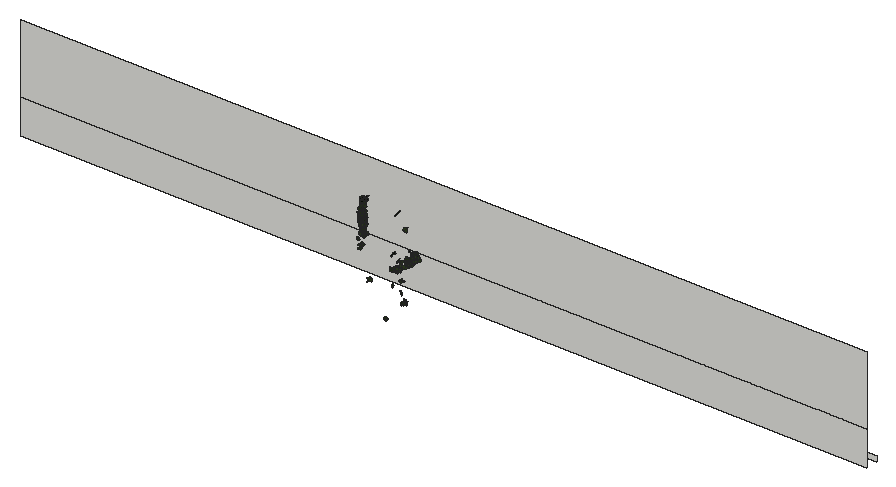
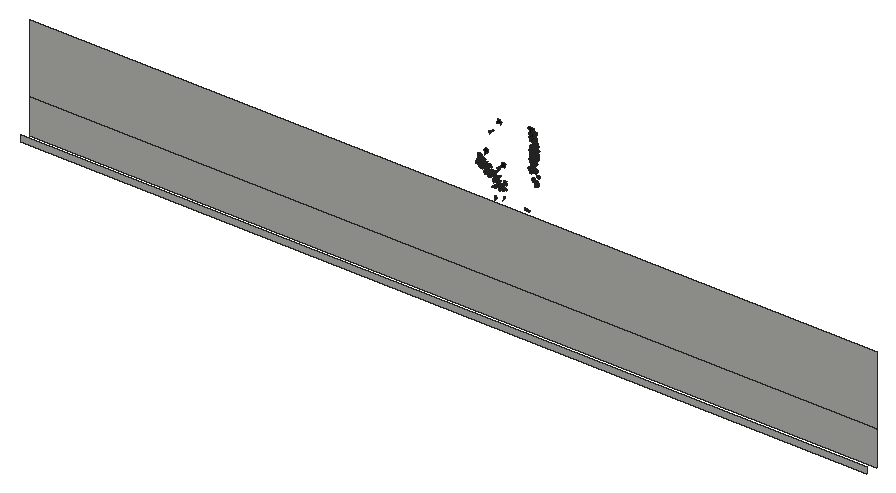
# SketchUp Ruby script. Lengths in inches.
U = 1.inch
M = Sketchup.active_model
def pt(a) = Geom::Point3d.new(a.map { |v| v * U })
def face(e, loops, mat)
  f = e.add_face(loops[0].map { |a| pt(a) })
  loops[1..].each { |l| e.add_face(l.map { |a| pt(a) }).erase! }
  f.material = f.back_material = mat if mat
  f
end
# faces: each face lists its corners as indices into pts; further lists are holes
def faces(e, pts, list, mat = nil) = list.each { |f| face(e, (f[0].is_a?(Array) ? f : [f]).map { |l| l.map { |i| pts[i] } }, mat) }
# xy, xz, yz: faces in a plane at the given z, y or x. An outline is a flat list of corners, or four numbers for a rectangle; further outlines are holes
def ring(l) = l.size == 4 ? [[l[0], l[1]], [l[2], l[1]], [l[2], l[3]], [l[0], l[3]]] : l.each_slice(2).to_a
def flat(e, list, mat, &to3) = list.each { |f| face(e, (f[0].is_a?(Array) ? f : [f]).map { |l| ring(l).map { |u, v| to3.(u, v) } }, mat) }
def xy(e, z, list, mat = nil) = flat(e, list, mat) { |x, y| [x, y, z] }
def xz(e, y, list, mat = nil) = flat(e, list, mat) { |x, z| [x, y, z] }
def yz(e, x, list, mat = nil) = flat(e, list, mat) { |y, z| [x, y, z] }
def lines(e, pts, list) = list.each { |a, b| e.add_line(pt(pts[a]), pt(pts[b])) }
# prism: a flat outline (further loops are holes) pulled along v
def prism(e, loops, v, mat = nil)
  f = face(e, loops, mat); d = Geom::Vector3d.new(v.map { |x| x * U })
  f.pushpull(f.normal.samedirection?(d) ? d.length : -d.length)
end
def box(e, o, s, mat = nil) = prism(e, [[o, [o[0] + s[0], o[1], o[2]], [o[0] + s[0], o[1] + s[1], o[2]], [o[0], o[1] + s[1], o[2]]]], [0, 0, s[2]], mat)
def at(x, y, z, deg = 0) = Geom::Transformation.translation(pt([x, y, z])) * Geom::Transformation.rotation(ORIGIN, Z_AXIS, deg.degrees)
def axes(o, x, y, z) = Geom::Transformation.new([*x, 0, *y, 0, *z, 0, *pt(o).to_a, 1])
def part(name) = M.definitions.add(name)
# library, detail: a bought-in or finely detailed component or shape, given as its bounding box
def library(name, o, s) = part(name).tap { |d| box(d.entities, o, s) }
def detail(e, o, s) = box(e.add_group.entities, o, s)
def put(e, d, t, mat = nil) = e.add_instance(d, t).tap { |i| i.material = mat if mat }
def group(e, t, mat = nil) = e.add_group.tap { |g| g.transformation = t; g.material = mat if mat }.entities
root = M.entities
M.materials.add("1026 AP 7946 SUNNY SIDE UP").color = [254, 231, 186]
M.materials.add("efeu1").color = [18, 25, 13]
M.materials.add("efeu2").color = [43, 57, 29]
c1 = part("ivyleaf_10")
p = [[0,0.5,-0.03],[-0.0625,2.02,-0.43],[-0.19,2.01,-0.46],[-0.54,1.05,-0.29],[-0.52,0.625,-0.18],[-0.83,0.76,-0.28],
  [-1.16,0.64,-0.33],[-1.15,0.33,-0.24],[-0.77,-0.39,0.02],[-0.3,-0.51,0.16],[0.04,-0.48,0.23],[-0.02,2.01,-0.4375],
  [-0.06,2.01,-0.43],[0.04,-0.49,0.23],[0.67,-0.49,0.14],[1.38,0.36,-0.2],[1.375,0.51,-0.24],[0.81,0.65,-0.19],
  [0.62,0.59,-0.15],[0.6,1.09,-0.28],[0.5,1.23,-0.31]]
faces(c1.entities,p,[[0,1,2,3,4,5,6,7,8,9,10],[11,12,0,13,14,15,16,17,18,19,20]],"efeu2")
c2 = part("ivyleaf_9")
p = [[1.54,2.16,1.25],[1.36,2.04,1.19],[-0.21,0.99,0.68],[-0.71,1.11,0.82],[-0.85,0.86,0.67],[-0.8,0.17,0.21],
  [-0.9,-0.01,0.1],[-0.67,-0.16,-0.02],[-0.08,-0.08,-0.05],[-0.03,-0.6,-0.4],[0.65,-0.88,-0.66],[0.83,-0.6,-0.49],
  [1.29,-0.42,-0.43],[1.8125,-0.07,-0.26],[1.21,0.44,0.15]]
faces(c2.entities,p,[[0,1,2,3,4,5,6,7,8,9,10,11,12,13,14]],"efeu1")
xz(root,227,[[30,246,177,252],[30,252,177,264]])
xz(root,229,[[30,246,177,247]])
put(root,c1,axes([99.8,213.53,264.95],[-0.08573,0.18101,-0.009],[-0.00321,-0.0117,-0.20128],[-0.3078,-0.05029,0.0046]),"1026 AP 7946 SUNNY SIDE UP")
put(root,c1,axes([99.82,213.11,265.17],[-0.13525,0.17041,-0.00934],[-0.00346,-0.01302,-0.20142],[-0.28985,-0.07936,0.00676]),"1026 AP 7946 SUNNY SIDE UP")
put(root,c1,axes([99.62,213.2,260.61],[0.00688,-0.00404,0.19077],[0.29489,-0.04004,-0.00576],[0.06813,0.17374,0.00566]),"1026 AP 7946 SUNNY SIDE UP")
put(root,c1,axes([99.73,213.47,263.92],[0.09541,0.05576,-0.17419],[0.16528,0.13172,0.08579],[0.2421,-0.1119,0.01008]),"1026 AP 7946 SUNNY SIDE UP")
put(root,c1,axes([99.8125,213.33,263.53],[0.16968,0.1463,-0.03606],[-0.01785,-0.03583,-0.18981],[-0.25497,0.09987,-0.0107]),"1026 AP 7946 SUNNY SIDE UP")
put(root,c1,axes([100.1,213.17,263.67],[-0.03089,0.023,0.19132],[-0.29433,0.04551,-0.02458],[-0.08132,-0.17346,0.01629]),"1026 AP 7946 SUNNY SIDE UP")
put(root,c1,axes([100,213.125,264.22],[0.18705,-0.12329,-0.09138],[-0.10102,0.05909,-0.17613],[0.23196,0.12515,-0.00302]),"1026 AP 7946 SUNNY SIDE UP")
put(root,c1,axes([99.92,213.55,265.11],[-0.22966,-0.12001,-0.04682],[0.08561,0.00591,-0.19115],[0.19823,-0.14159,0.0283]),"1026 AP 7946 SUNNY SIDE UP")
put(root,c1,axes([99.96,213.55,264.52],[0.00212,0.17404,0.05604],[-0.07134,0.04899,-0.18048],[-0.29904,-0.01045,0.04345]),"1026 AP 7946 SUNNY SIDE UP")
put(root,c1,axes([99.96,213.58,263.82],[0.14893,-0.15282,0.01887],[0.00536,-0.02078,-0.18876],[0.26148,0.08746,-0.00687]),"1026 AP 7946 SUNNY SIDE UP")
put(root,c1,axes([99.98,213.3125,263.88],[0.0121,0.13669,-0.11707],[-0.05804,-0.10803,-0.14612],[-0.29336,0.02701,0.02408]),"1026 AP 7946 SUNNY SIDE UP")
put(root,c1,axes([100.11,213.24,263.96],[-0.23706,0.08116,0.09126],[-0.16438,-0.00676,-0.16509],[-0.11128,-0.16292,0.04947]),"1026 AP 7946 SUNNY SIDE UP")
put(root,c1,axes([99.96,213.56,263.99],[0.01126,0.15169,0.10111],[-0.01801,0.09271,-0.1607],[-0.30103,0.00013,0.0134]),"1026 AP 7946 SUNNY SIDE UP")
put(root,c1,axes([100.09,213.17,263.96],[0.26296,-0.01763,-0.10344],[-0.16562,-0.01098,-0.16586],[0.01547,0.18212,-0.01744]),"1026 AP 7946 SUNNY SIDE UP")
put(root,c1,axes([99.98,213.55,265.05],[0.0413,0.18007,-0.03465],[-0.03651,-0.03197,-0.19415],[-0.30916,0.02783,0.0183]),"1026 AP 7946 SUNNY SIDE UP")
put(root,c1,axes([99.96,213.3125,264.65],[-0.21143,-0.10896,-0.08139],[0.10849,0.04001,-0.17622],[0.19617,-0.13956,0.00973]),"1026 AP 7946 SUNNY SIDE UP")
put(root,c1,axes([100.05,213.16,264.73],[-0.29522,-0.07091,0.01055],[-0.00665,-0.01883,-0.2006],[0.12158,-0.17322,0.01464]),"1026 AP 7946 SUNNY SIDE UP")
put(root,c1,axes([100.01,213.58,265.22],[0.2454,-0.11687,0.00366],[-0.00906,-0.01445,-0.1986],[0.19836,0.14392,-0.01361]),"1026 AP 7946 SUNNY SIDE UP")
put(root,c1,axes([100.05,213.1875,264.34],[0.21336,-0.13975,-0.01992],[-0.03616,0.00335,-0.20065],[0.23618,0.12676,-0.01273]),"1026 AP 7946 SUNNY SIDE UP")
put(root,c1,axes([99.99,213.13,259.1],[-0.13186,-0.14776,0.0643],[0.03866,0.05801,0.17939],[-0.26924,0.08069,-0.00573]),"1026 AP 7946 SUNNY SIDE UP")
put(root,c1,axes([99.84,213.53,263.92],[-0.07983,-0.0293,0.18382],[0.26154,0.07681,0.06015],[-0.1393,0.16101,0.00759]),"1026 AP 7946 SUNNY SIDE UP")
put(root,c1,axes([100.16,213.22,263.12],[0.16699,-0.05763,-0.14715],[-0.1384,0.11603,-0.11356],[0.21039,0.12207,0.04209]),"1026 AP 7946 SUNNY SIDE UP")
put(root,c1,axes([99.92,213.3,262.71],[-0.01351,-0.07917,-0.17288],[0.16678,-0.13616,0.06481],[-0.25383,-0.08525,0.05179]),"1026 AP 7946 SUNNY SIDE UP")
put(root,c1,axes([100.05,213.29,265.82],[-0.01285,-0.18492,-0.06657],[0.07676,0.0565,-0.19248],[0.32085,-0.02092,0.04338]),"1026 AP 7946 SUNNY SIDE UP")
put(root,c1,axes([100.12,213.17,265.4],[-0.22306,-0.14248,-0.00525],[0.01779,-0.00553,-0.20722],[0.24127,-0.13132,0.01042]),"1026 AP 7946 SUNNY SIDE UP")
put(root,c1,axes([100.02,213.36,266.59],[-0.26377,0.08331,-0.08758],[0.09825,-0.06535,-0.18737],[-0.17363,-0.16354,0.02702]),"1026 AP 7946 SUNNY SIDE UP")
put(root,c1,axes([100.03,213.17,259.82],[-0.25598,-0.07031,-0.07507],[0.13654,-0.01444,-0.17214],[0.09696,-0.16528,0.04422]),"1026 AP 7946 SUNNY SIDE UP")
put(root,c1,axes([100.18,213.21,263.19],[-0.22695,-0.10627,0.04612],[-0.04488,-0.03799,-0.18285],[0.19032,-0.13568,0.01188]),"1026 AP 7946 SUNNY SIDE UP")
put(root,c1,axes([100.02,213.28,261.32],[-0.18875,-0.03234,0.14969],[0.21325,0.06469,0.1235],[-0.11924,0.16688,-0.01609]),"1026 AP 7946 SUNNY SIDE UP")
put(root,c1,axes([100.14,213.51,264.78],[0.05697,0.18388,-0.02115],[-0.00004,-0.02251,-0.20037],[-0.31439,0.03332,-0.00381]),"1026 AP 7946 SUNNY SIDE UP")
put(root,c1,axes([100.04,213.125,263.24],[-0.12162,-0.09602,-0.14303],[0.25004,0.02483,-0.1043],[0.1205,-0.14843,0.07207]),"1026 AP 7946 SUNNY SIDE UP")
put(root,c1,axes([100.24,213.39,267.2],[-0.05572,-0.20079,0.01294],[0.00401,-0.01528,-0.21797],[0.34174,-0.03256,0.00467]),"1026 AP 7946 SUNNY SIDE UP")
put(root,c1,axes([100.22,213.24,266.23],[-0.28996,0.09434,-0.02977],[0.02583,-0.03218,-0.20819],[-0.16556,-0.17025,0.01966]),"1026 AP 7946 SUNNY SIDE UP")
put(root,c1,axes([100.26,213.28,265.1],[0.15146,-0.16796,-0.00621],[-0.01712,-0.00127,-0.20337],[0.28466,0.08929,-0.00893]),"1026 AP 7946 SUNNY SIDE UP")
put(root,c1,axes([100.23,213.25,265.89],[-0.23245,0.13793,-0.01368],[0.00065,-0.02011,-0.20783],[-0.23545,-0.13623,0.01294]),"1026 AP 7946 SUNNY SIDE UP")
put(root,c1,axes([100.2,213.09,262.33],[-0.0186,-0.04099,-0.18598],[0.10384,0.16208,-0.04295],[0.28371,-0.06201,0.00352]),"1026 AP 7946 SUNNY SIDE UP")
put(root,c1,axes([100.2,213.26,263.27],[0.05277,0.12995,0.12927],[0.01746,0.11934,-0.14067],[-0.29866,0.02994,0.01462]),"1026 AP 7946 SUNNY SIDE UP")
put(root,c1,axes([100.28,213.06,262.64],[0.03778,-0.03056,-0.20052],[0.01439,0.18816,-0.02923],[0.32117,-0.00484,0.0249]),"1026 AP 7946 SUNNY SIDE UP")
put(root,c1,axes([100.3125,213.29,263.67],[0.01894,-0.1781,-0.01212],[-0.00558,0.00881,-0.1909],[0.30266,0.01131,-0.00276]),"1026 AP 7946 SUNNY SIDE UP")
put(root,c1,axes([100.33,213.26,262.83],[0.11148,-0.15735,-0.05242],[-0.04438,0.03986,-0.18176],[0.27517,0.07018,-0.00808]),"1026 AP 7946 SUNNY SIDE UP")
put(root,c1,axes([100.31,213.54,263.46],[0.12116,-0.12155,0.11326],[-0.08101,0.09638,0.15211],[-0.26312,-0.08564,0.00532]),"1026 AP 7946 SUNNY SIDE UP")
put(root,c1,axes([100.36,213.08,261.33],[0.03254,0.1756,-0.0385],[-0.01151,0.03915,0.18931],[0.30486,-0.01726,0.01126]),"1026 AP 7946 SUNNY SIDE UP")
put(root,c1,axes([100.41,213.21,263.65],[-0.25777,0.10349,0.03786],[-0.064,0.00481,-0.19583],[-0.1735,-0.15554,0.016]),"1026 AP 7946 SUNNY SIDE UP")
put(root,c1,axes([100.3,213.55,263.6],[0.24114,0.06526,0.09295],[0.13867,0.02787,-0.16677],[-0.11975,0.16368,-0.00595]),"1026 AP 7946 SUNNY SIDE UP")
put(root,c1,axes([100.5,213.21,260.09],[-0.30075,0.02438,-0.00035],[-0.00304,-0.01776,-0.19075],[-0.0413,-0.17628,0.01664]),"1026 AP 7946 SUNNY SIDE UP")
put(root,c1,axes([100.51,213.125,265.85],[-0.03829,-0.20467,-0.07042],[0.04974,0.05992,-0.21839],[0.36016,-0.03003,0.02267]),"1026 AP 7946 SUNNY SIDE UP")
put(root,c2,axes([100.47,213.05,267.2],[0.2335,0.17699,0.02866],[0.04404,0.01076,-0.23937],[-0.3001,0.13929,-0.01283]),"1026 AP 7946 SUNNY SIDE UP")
put(root,c1,axes([100.51,213.12,266],[-0.22221,-0.16159,-0.06915],[0.12202,0.0206,-0.21797],[0.2676,-0.14358,0.04197]),"1026 AP 7946 SUNNY SIDE UP")
put(root,c1,axes([100.63,213.3125,261.9375],[0.20373,-0.12375,-0.06636],[-0.08127,0.03758,-0.18384],[0.21915,0.12898,-0.00649]),"1026 AP 7946 SUNNY SIDE UP")
put(root,c1,axes([100.55,213.58,263.38],[-0.04647,-0.1594,-0.07776],[0.10679,0.05758,-0.16457],[0.27597,-0.04912,0.05059]),"1026 AP 7946 SUNNY SIDE UP")
put(root,c1,axes([100.59,213.2,264.56],[-0.12568,-0.18895,-0.03934],[0.07714,0.01846,-0.21373],[0.31672,-0.07947,0.03644]),"1026 AP 7946 SUNNY SIDE UP")
put(root,c1,axes([100.73,213.25,262.96],[-0.27297,-0.05676,0.08744],[-0.11633,-0.05121,-0.18162],[0.12379,-0.17329,0.02214]),"1026 AP 7946 SUNNY SIDE UP")
put(root,c2,axes([100.58,213.27,266.65],[0.2053,0.17402,0.01628],[0.02611,0.00504,-0.22656],[-0.29507,0.12152,-0.00873]),"1026 AP 7946 SUNNY SIDE UP")
put(root,c1,axes([100.6,213.2,267.34],[-0.33728,-0.08153,-0.0468],[0.0805,-0.00375,-0.22887],[0.13386,-0.20318,0.01971]),"1026 AP 7946 SUNNY SIDE UP")
put(root,c1,axes([100.61,213.32,264.375],[-0.26385,0.08434,-0.04903],[0.01507,-0.07604,-0.17895],[-0.16312,-0.14344,0.06278]),"1026 AP 7946 SUNNY SIDE UP")
put(root,c1,axes([100.66,213.32,261.95],[-0.27978,0.08015,0.00689],[-0.03009,-0.02427,-0.19398],[-0.13301,-0.16311,0.02938]),"1026 AP 7946 SUNNY SIDE UP")
put(root,c1,axes([100.68,213.29,264.17],[-0.03298,-0.17704,0.08764],[-0.00653,-0.08423,-0.19178],[0.3327,-0.0192,0.00493]),"1026 AP 7946 SUNNY SIDE UP")
put(root,c1,axes([100.69,213.29,262.27],[-0.04499,-0.15422,0.1048],[-0.02046,-0.09926,-0.16886],[0.31126,-0.02882,0.00405]),"1026 AP 7946 SUNNY SIDE UP")
put(root,c1,axes([100.7,213.26,265.25],[-0.3069,-0.09078,0.01342],[-0.00872,-0.02025,-0.2162],[0.15561,-0.18017,0.01435]),"1026 AP 7946 SUNNY SIDE UP")
put(root,c1,axes([100.65,213.26,265.13],[0.08984,0.19186,-0.0504],[-0.04783,-0.04351,-0.21306],[-0.33297,0.05802,0.01701]),"1026 AP 7946 SUNNY SIDE UP")
put(root,c2,axes([100.6,213.2,266.92],[0.24939,0.14083,0.08258],[0.0465,0.07858,-0.21345],[-0.26708,0.14518,0.03995]),"1026 AP 7946 SUNNY SIDE UP")
put(root,c1,axes([100.71,213.22,266.11],[0.31918,0.08631,-0.0536],[-0.08619,-0.01195,-0.2214],[-0.14694,0.1945,0.01344]),"1026 AP 7946 SUNNY SIDE UP")
put(root,c1,axes([100.67,213.33,264.26],[-0.00056,-0.1444,0.14045],[0.00033,0.13308,0.15644],[-0.33334,0.00037,-0.00008]),"1026 AP 7946 SUNNY SIDE UP")
put(root,c1,axes([100.76,213.37,261.33],[-0.14655,-0.15182,0.02679],[-0.00599,-0.029,-0.187],[0.2617,-0.08568,0.01072]),"1026 AP 7946 SUNNY SIDE UP")
put(root,c1,axes([100.71,213.18,266.23],[0.02929,0.206,0.0532],[-0.04933,0.04903,-0.21792],[-0.35527,0.01017,0.03464]),"1026 AP 7946 SUNNY SIDE UP")
put(root,c1,axes([100.8,213.24,263.95],[-0.33038,0.02541,0.03441],[-0.06092,-0.03369,-0.20671],[-0.03264,-0.19431,0.0375]),"1026 AP 7946 SUNNY SIDE UP")
put(root,c1,axes([100.71,213.43,262.26],[-0.14821,0.12742,-0.09223],[0.00134,-0.10046,-0.15829],[-0.26268,-0.0724,0.05123]),"1026 AP 7946 SUNNY SIDE UP")
put(root,c1,axes([100.76,213.17,267.02],[-0.36795,-0.03167,0.00632],[0.0067,-0.06854,-0.22376],[0.05441,-0.20573,0.07032]),"1026 AP 7946 SUNNY SIDE UP")
put(root,c1,axes([100.73,213.13,261.45],[0.00762,-0.18561,-0.0547],[0.05096,0.04877,-0.19544],[0.32172,-0.00333,0.03225]),"1026 AP 7946 SUNNY SIDE UP")
put(root,c1,axes([100.73,213.16,264.2],[0.33774,0.02828,-0.03422],[-0.05361,-0.00758,-0.21523],[-0.04943,0.20143,-0.00042]),"1026 AP 7946 SUNNY SIDE UP")
put(root,c1,axes([100.71,213.23,264.53],[-0.06186,0.18836,-0.04216],[0.00267,-0.04228,-0.20587],[-0.32753,-0.03592,0.00628]),"1026 AP 7946 SUNNY SIDE UP")
put(root,c1,axes([100.76,213.25,263.79],[0.07543,-0.18454,0.04906],[0.02667,-0.04581,-0.20379],[0.32268,0.04692,0.00538]),"1026 AP 7946 SUNNY SIDE UP")
put(root,c1,axes([100.8,213.37,262.99],[-0.20668,-0.13708,0.00757],[0.00558,-0.01475,-0.19605],[0.23312,-0.12118,0.01141]),"1026 AP 7946 SUNNY SIDE UP")
put(root,c1,axes([100.72,213.23,262.99],[0.27726,0.09669,-0.02185],[-0.01858,-0.02391,-0.20291],[-0.16718,0.16301,-0.01368]),"1026 AP 7946 SUNNY SIDE UP")
put(root,c2,axes([100.8125,213.16,267.01],[0.15282,0.19745,-0.0266],[-0.00698,-0.02824,-0.23256],[-0.33833,0.08977,-0.00722]),"1026 AP 7946 SUNNY SIDE UP")
put(root,c1,axes([100.78,213.23,265.3],[-0.06627,0.20305,-0.01173],[-0.01508,-0.01553,-0.22123],[-0.34513,-0.03831,0.01192]),"1026 AP 7946 SUNNY SIDE UP")
put(root,c1,axes([100.79,213.28,263.37],[0.04033,0.18538,-0.05285],[-0.04142,-0.04885,-0.1999],[-0.32409,0.02931,0.01897]),"1026 AP 7946 SUNNY SIDE UP")
put(root,c1,axes([100.72,213.19,264.73],[-0.25865,-0.07372,-0.12725],[0.20399,0.01818,-0.17818],[0.11875,-0.19179,0.02893]),"1026 AP 7946 SUNNY SIDE UP")
put(root,c1,axes([100.72,213.17,267.33],[0.34741,0.02722,0.07086],[0.11215,0.00238,-0.2209],[-0.04523,0.21497,-0.00347]),"1026 AP 7946 SUNNY SIDE UP")
put(root,c1,axes([100.8125,213.34,262.55],[0.228,-0.10498,0.05928],[0.06302,-0.04443,-0.18271],[0.19252,0.13887,-0.01039]),"1026 AP 7946 SUNNY SIDE UP")
put(root,c1,axes([100.78,213.28,263.09],[0.12767,0.15598,0.09251],[0.05991,0.07665,-0.18431],[-0.29502,0.08307,0.00261]),"1026 AP 7946 SUNNY SIDE UP")
put(root,c1,axes([100.85,213.34,263.23],[0.20384,0.14238,-0.03471],[-0.02269,-0.03349,-0.19951],[-0.24756,0.1203,-0.0103]),"1026 AP 7946 SUNNY SIDE UP")
put(root,c1,axes([100.91,213.32,263.68],[-0.22974,0.13704,0.00566],[-0.01782,-0.00545,-0.20592],[-0.23202,-0.13527,0.0102]),"1026 AP 7946 SUNNY SIDE UP")
put(root,c1,axes([100.82,213.38,261.75],[-0.19932,-0.08305,-0.11361],[0.16998,0.0383,-0.15171],[0.15091,-0.15282,0.02082]),"1026 AP 7946 SUNNY SIDE UP")
put(root,c1,axes([100.92,213.26,264.42],[0.33259,0.0232,-0.02253],[-0.03301,-0.01679,-0.2109],[-0.04212,0.19637,-0.01257]),"1026 AP 7946 SUNNY SIDE UP")
put(root,c2,axes([100.99,212.95,267.61],[0.16376,0.21399,0.10037],[0.0109,0.10242,-0.24179],[-0.36877,0.09806,0.03742]),"1026 AP 7946 SUNNY SIDE UP")
put(root,c1,axes([100.82,213.38,261.82],[-0.14749,-0.02096,-0.16607],[0.26385,-0.02984,-0.08946],[-0.02732,-0.17503,0.03259]),"1026 AP 7946 SUNNY SIDE UP")
put(root,c1,axes([101.75,213.24,254.98],[-0.37461,0.09672,0.05825],[-0.18068,-0.1551,-0.1731],[-0.04953,-0.16573,0.19087]),"1026 AP 7946 SUNNY SIDE UP")
put(root,c1,axes([104.73,213.08,249.91],[0.11614,-0.08669,-0.18108],[-0.21873,0.10839,-0.11498],[0.2161,0.1563,-0.01907]),"1026 AP 7946 SUNNY SIDE UP")
put(root,c1,axes([104.94,213.92,257.42],[0.2611,-0.11138,0.03878],[0.06338,-0.00842,-0.20544],[0.17401,0.1702,0.01664]),"1026 AP 7946 SUNNY SIDE UP")
put(root,c1,axes([105.34,213.93,257.71],[-0.23358,0.12624,-0.06654],[0.02097,-0.08166,-0.19437],[-0.22251,-0.14022,0.05153]),"1026 AP 7946 SUNNY SIDE UP")
put(root,c1,axes([105.59,213.1,257.86],[-0.24893,0.08041,0.16639],[-0.25236,0.0341,-0.17985],[-0.1282,-0.22325,0.03095]),"1026 AP 7946 SUNNY SIDE UP")
put(root,c1,axes([105.55,213.91,257.65],[-0.20881,-0.10694,0.1191],[-0.107,-0.09827,-0.17385],[0.2241,-0.14657,0.02796]),"1026 AP 7946 SUNNY SIDE UP")
put(root,c1,axes([105.46,214.17,257.32],[-0.15778,0.17467,-0.02479],[0.0103,-0.02511,-0.20756],[-0.27728,-0.10033,0.00639]),"1026 AP 7946 SUNNY SIDE UP")
put(root,c1,axes([105.62,213.18,255.28],[-0.0145,0.06289,0.19903],[-0.11432,0.17919,-0.06274],[-0.29775,-0.07186,0.01439]),"1026 AP 7946 SUNNY SIDE UP")
put(root,c1,axes([105.45,214,257.24],[-0.22549,-0.08329,-0.12235],[0.20522,-0.00263,-0.16111],[0.09814,-0.18588,0.0558]),"1026 AP 7946 SUNNY SIDE UP")
put(root,c1,axes([105.89,214.05,257.65],[-0.30584,0.06508,0.02196],[-0.04396,-0.01804,-0.20972],[-0.09811,-0.1948,0.02549]),"1026 AP 7946 SUNNY SIDE UP")
put(root,c2,axes([105.91,212.94,260.4],[-0.06282,0.05516,-0.24528],[-0.15045,0.21881,0.06995],[0.35414,0.10274,-0.01379]),"1026 AP 7946 SUNNY SIDE UP")
put(root,c1,axes([106.13,213.95,258.15],[-0.1523,-0.16052,0.09545],[-0.06758,-0.0833,-0.19354],[0.28423,-0.10582,0.00513]),"1026 AP 7946 SUNNY SIDE UP")
put(root,c1,axes([106.17,213.77,258.1],[0.22998,-0.13922,-0.01627],[-0.02673,0.00388,-0.2078],[0.21856,0.14698,-0.00829]),"1026 AP 7946 SUNNY SIDE UP")
put(root,c1,axes([106.53,214.21,258.18],[-0.16036,-0.10558,0.1526],[-0.01213,-0.16775,-0.12911],[0.28653,-0.06619,0.07994]),"1026 AP 7946 SUNNY SIDE UP")
put(root,c1,axes([106.5,214.05,258.53],[-0.22007,0.14625,-0.01709],[0.00497,-0.02104,-0.20828],[-0.23154,-0.13946,0.01177]),"1026 AP 7946 SUNNY SIDE UP")
put(root,c1,axes([106.49,213.41,257.83],[0.31659,0.0246,-0.00444],[-0.003,-0.02088,-0.20802],[-0.0392,0.2003,-0.01994]),"1026 AP 7946 SUNNY SIDE UP")
put(root,c2,axes([106.61,212.93,266.82],[-0.17334,0.16391,-0.16267],[-0.1124,0.14272,0.20368],[0.34083,0.13043,-0.01556]),"1026 AP 7946 SUNNY SIDE UP")
put(root,c1,axes([106.64,213.96,259.08],[0.06945,0.16615,-0.11463],[-0.1011,-0.09709,-0.17474],[-0.2986,0.07152,0.03251]),"1026 AP 7946 SUNNY SIDE UP")
put(root,c1,axes([106.59,213.15,258.33],[0.22378,0.14494,-0.00076],[0.01498,-0.01154,-0.20876],[-0.22742,0.14186,-0.0145]),"1026 AP 7946 SUNNY SIDE UP")
put(root,c1,axes([106.64,213.125,259.42],[0.09142,-0.17589,0.16644],[-0.03926,0.16192,0.19064],[-0.37456,-0.0599,0.02064]),"1026 AP 7946 SUNNY SIDE UP")
put(root,c1,axes([106.79,214,258.3],[0.02959,-0.20316,0.04936],[0.05925,-0.04516,-0.20778],[0.32324,0.02687,0.03357]),"1026 AP 7946 SUNNY SIDE UP")
put(root,c1,axes([107.24,213.16,253.03],[-0.05424,0.08162,0.21194],[-0.16386,0.17717,-0.08958],[-0.30626,-0.10924,0.01039]),"1026 AP 7946 SUNNY SIDE UP")
put(root,c1,axes([107.1,213.17,254.86],[-0.20856,0.14461,-0.10629],[0.09114,-0.08757,-0.20211],[-0.26484,-0.14401,0.01415]),"1026 AP 7946 SUNNY SIDE UP")
put(root,c1,axes([107.07,213.16,256.625],[0.06009,0.02038,0.21186],[0.21138,0.15624,-0.0408],[-0.24657,0.13891,0.01666]),"1026 AP 7946 SUNNY SIDE UP")
put(root,c1,axes([107.32,214.03,259.26],[-0.10991,0.20031,-0.03953],[0.01677,-0.03812,-0.21877],[-0.3206,-0.07066,0.00211]),"1026 AP 7946 SUNNY SIDE UP")
put(root,c1,axes([107.29,214.02,258.57],[-0.12748,-0.13699,0.14366],[0.20585,0.07512,0.15401],[-0.22944,0.14351,0.05835]),"1026 AP 7946 SUNNY SIDE UP")
put(root,c1,axes([107.61,213.88,259.26],[0.2841,-0.10573,0.01086],[0.00771,-0.01365,-0.21553],[0.167,0.18051,-0.00852]),"1026 AP 7946 SUNNY SIDE UP")
put(root,c1,axes([107.8125,214.03,259.49],[0.08558,-0.02858,-0.21595],[-0.20596,0.16522,-0.05732],[0.26092,0.13979,0.02559]),"1026 AP 7946 SUNNY SIDE UP")
put(root,c1,axes([107.85,213.94,259.97],[-0.12516,-0.04763,0.20088],[-0.21889,-0.13843,-0.09405],[0.22797,-0.15907,0.01999]),"1026 AP 7946 SUNNY SIDE UP")
put(root,c1,axes([107.73,213.27,258.91],[0.31293,0.01974,-0.06113],[-0.08863,-0.02995,-0.20481],[-0.04296,0.20553,-0.02274]),"1026 AP 7946 SUNNY SIDE UP")
put(root,c1,axes([107.82,214.04,259.1875],[-0.1346,-0.1981,0.00822],[0.00633,-0.01165,-0.22222],[0.31175,-0.08529,0.00806]),"1026 AP 7946 SUNNY SIDE UP")
put(root,c1,axes([107.71,213.17,253.34],[0.04381,0.1792,0.14],[0.03502,0.13304,-0.18605],[-0.35094,0.03565,-0.00108]),"1026 AP 7946 SUNNY SIDE UP")
put(root,c1,axes([107.73,214.05,259.14],[0.20309,-0.15376,0.08061],[0.09567,-0.05203,-0.20679],[0.25451,0.14225,0.01341]),"1026 AP 7946 SUNNY SIDE UP")
put(root,c1,axes([107.82,213.23,253.77],[-0.30273,0.09394,-0.07492],[0.08666,-0.0532,-0.21979],[-0.16606,-0.19901,0.02189]),"1026 AP 7946 SUNNY SIDE UP")
put(root,c1,axes([107.85,214.07,259],[0.33662,-0.00315,0.01978],[0.02961,-0.02036,-0.21973],[0.00777,0.21398,-0.01935]),"1026 AP 7946 SUNNY SIDE UP")
put(root,c1,axes([107.97,214.34,259.26],[-0.30174,0.09726,0.01734],[-0.04248,-0.01758,-0.21988],[-0.14913,-0.19178,0.02754]),"1026 AP 7946 SUNNY SIDE UP")
put(root,c1,axes([107.93,212.98,264.8],[0.16547,0.05738,-0.23985],[0.14961,0.22375,0.10228],[0.34663,-0.12396,0.07035]),"1026 AP 7946 SUNNY SIDE UP")
put(root,c1,axes([107.98,214.18,259.26],[0.03431,0.21042,-0.04753],[-0.00202,-0.04745,-0.21818],[-0.33913,0.02157,-0.00351]),"1026 AP 7946 SUNNY SIDE UP")
put(root,c1,axes([108.04,214.14,259.05],[0.33808,0.00468,0.01902],[0.0296,-0.02209,-0.22048],[-0.00433,0.21467,-0.02183]),"1026 AP 7946 SUNNY SIDE UP")
put(root,c1,axes([108.33,214.11,260.09],[-0.19028,0.08085,0.17186],[-0.27109,0.02273,-0.14044],[-0.10538,-0.20446,0.05095]),"1026 AP 7946 SUNNY SIDE UP")
put(root,c1,axes([108.25,214.08,260.11],[-0.02698,-0.20992,0.02167],[0.00539,-0.02257,-0.21705],[0.33188,-0.0167,0.00529]),"1026 AP 7946 SUNNY SIDE UP")
put(root,c1,axes([108.45,213.54,259.36],[0.26199,0.131,-0.01629],[-0.00519,-0.02252,-0.21788],[-0.20755,0.16592,-0.01512]),"1026 AP 7946 SUNNY SIDE UP")
put(root,c1,axes([108.57,214.1,260.89],[0.31529,-0.07801,-0.04473],[-0.07586,-0.00613,-0.22044],[0.11772,0.20498,-0.02225]),"1026 AP 7946 SUNNY SIDE UP")
put(root,c1,axes([108.6,214.16,260.1875],[0.15034,0.18441,-0.0494],[-0.01454,-0.05026,-0.21376],[-0.29967,0.09495,-0.01441]),"1026 AP 7946 SUNNY SIDE UP")
put(root,c1,axes([108.66,214.125,260.29],[0.29867,0.09869,-0.01485],[-0.00739,-0.02332,-0.21983],[-0.15678,0.1891,-0.01793]),"1026 AP 7946 SUNNY SIDE UP")
put(root,c1,axes([108.72,214.32,259.74],[0.3381,0.0235,-0.03609],[-0.05491,-0.0042,-0.22286],[-0.03753,0.21784,0.00088]),"1026 AP 7946 SUNNY SIDE UP")
put(root,c1,axes([108.8,214.11,260.17],[-0.31333,0.0776,0.00298],[-0.03827,-0.05603,-0.21146],[-0.11592,-0.19124,0.06176]),"1026 AP 7946 SUNNY SIDE UP")
put(root,c1,axes([108.84,213.3125,259.71],[-0.08431,-0.1664,0.12644],[-0.01526,-0.1256,-0.17915],[0.32565,-0.04897,0.02434]),"1026 AP 7946 SUNNY SIDE UP")
put(root,c2,axes([108.82,213.09,261.66],[0.30913,-0.05286,-0.16608],[-0.2494,0.029,-0.20929],[0.0934,0.25239,-0.00918]),"1026 AP 7946 SUNNY SIDE UP")
put(root,c1,axes([108.98,213.74,260.02],[0.06666,0.21074,0.02332],[-0.00404,0.02237,-0.22121],[-0.33305,0.04191,0.00735]),"1026 AP 7946 SUNNY SIDE UP")
put(root,c1,axes([109.08,214.06,261.14],[-0.26067,-0.10364,-0.09975],[0.15297,0.02408,-0.1992],[0.16142,-0.19017,0.02768]),"1026 AP 7946 SUNNY SIDE UP")
put(root,c1,axes([109.18,214.16,260.62],[0.22054,0.16159,-0.03387],[-0.0131,-0.03736,-0.21987],[-0.25925,0.13935,-0.01771]),"1026 AP 7946 SUNNY SIDE UP")
put(root,c1,axes([109.26,214.14,260.85],[0.09218,-0.19024,-0.09047],[-0.0085,0.08867,-0.2036],[0.32865,0.05565,0.02011]),"1026 AP 7946 SUNNY SIDE UP")
put(root,c1,axes([109.12,214.05,261.28],[0.30119,-0.03635,0.10279],[0.16144,0.0092,-0.19913],[0.04383,0.21588,0.02709]),"1026 AP 7946 SUNNY SIDE UP")
put(root,c1,axes([109.39,214.34,260.17],[0.29905,-0.02353,-0.11596],[-0.17062,0.03452,-0.19634],[0.05923,0.21822,0.01988]),"1026 AP 7946 SUNNY SIDE UP")
